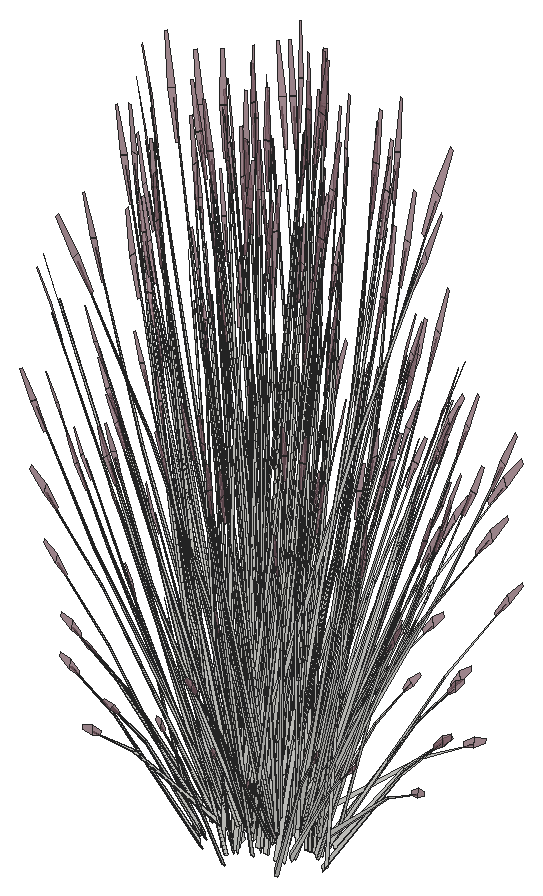
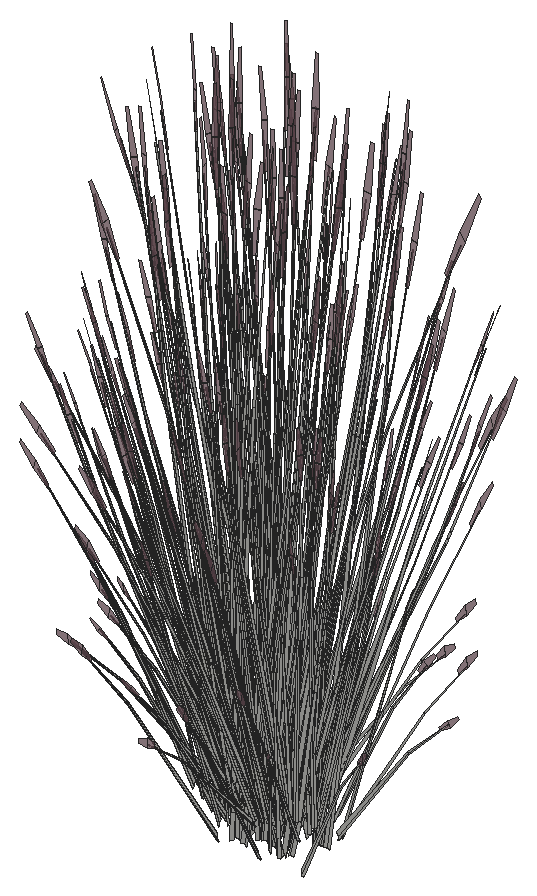
# SketchUp Ruby script. Lengths in inches.
U = 1.inch
M = Sketchup.active_model
def pt(a) = Geom::Point3d.new(a.map { |v| v * U })
def face(e, loops, mat)
  f = e.add_face(loops[0].map { |a| pt(a) })
  loops[1..].each { |l| e.add_face(l.map { |a| pt(a) }).erase! }
  f.material = f.back_material = mat if mat
  f
end
# faces: each face lists its corners as indices into pts; further lists are holes
def faces(e, pts, list, mat = nil) = list.each { |f| face(e, (f[0].is_a?(Array) ? f : [f]).map { |l| l.map { |i| pts[i] } }, mat) }
# xy, xz, yz: faces in a plane at the given z, y or x. An outline is a flat list of corners, or four numbers for a rectangle; further outlines are holes
def ring(l) = l.size == 4 ? [[l[0], l[1]], [l[2], l[1]], [l[2], l[3]], [l[0], l[3]]] : l.each_slice(2).to_a
def flat(e, list, mat, &to3) = list.each { |f| face(e, (f[0].is_a?(Array) ? f : [f]).map { |l| ring(l).map { |u, v| to3.(u, v) } }, mat) }
def xy(e, z, list, mat = nil) = flat(e, list, mat) { |x, y| [x, y, z] }
def xz(e, y, list, mat = nil) = flat(e, list, mat) { |x, z| [x, y, z] }
def yz(e, x, list, mat = nil) = flat(e, list, mat) { |y, z| [x, y, z] }
def lines(e, pts, list) = list.each { |a, b| e.add_line(pt(pts[a]), pt(pts[b])) }
# prism: a flat outline (further loops are holes) pulled along v
def prism(e, loops, v, mat = nil)
  f = face(e, loops, mat); d = Geom::Vector3d.new(v.map { |x| x * U })
  f.pushpull(f.normal.samedirection?(d) ? d.length : -d.length)
end
def box(e, o, s, mat = nil) = prism(e, [[o, [o[0] + s[0], o[1], o[2]], [o[0] + s[0], o[1] + s[1], o[2]], [o[0], o[1] + s[1], o[2]]]], [0, 0, s[2]], mat)
def at(x, y, z, deg = 0) = Geom::Transformation.translation(pt([x, y, z])) * Geom::Transformation.rotation(ORIGIN, Z_AXIS, deg.degrees)
def axes(o, x, y, z) = Geom::Transformation.new([*x, 0, *y, 0, *z, 0, *pt(o).to_a, 1])
def part(name) = M.definitions.add(name)
# library, detail: a bought-in or finely detailed component or shape, given as its bounding box
def library(name, o, s) = part(name).tap { |d| box(d.entities, o, s) }
def detail(e, o, s) = box(e.add_group.entities, o, s)
def put(e, d, t, mat = nil) = e.add_instance(d, t).tap { |i| i.material = mat if mat }
def group(e, t, mat = nil) = e.add_group.tap { |g| g.transformation = t; g.material = mat if mat }.entities
root = M.entities
M.materials.add("LightPink_Translucent").color = [144, 107, 117]
M.materials["LightPink_Translucent"].alpha = 0.75
c1 = part("blade")
p = [[2.15,0.21,22],[0,0.17,0],[0.09,0.45,0],[2.18,0.31,22],[2.29,0.31,22],[0.38,0.45,0],
  [2.48,0.24,33],[2.49,0.24,33],[2.48,0.22,33]]
faces(c1.entities,p,[[0,1,2,3],[4,5,2,3],[6,3,4,7],[8,0,3,6]])
c2 = part("seeds")
p = [[0.3,-0.1,1.38],[-0.01,-0.03,1.59],[-0.01,-0.03,0.03],[0.14,-0.07,-0.07],[0.29,-0.03,3],[0.15,0.01,3.11]]
faces(c2.entities,p,[[0,1,2,3],[1,0,4,5]],"LightPink_Translucent")
c3 = part("blade with seeds")
put(c3.entities,c1,at(0,0,0))
put(c3.entities,c2,axes([2.4,0.25,30.99],[1.5799,-0.05474,1.17369],[-0.12525,1.92788,0.29478],[-0.07173,-0.02425,1.56792]))
put(root,c3,axes([839.49,270.18,1.9375],[0.11478,-0.10046,0.85688],[0.28982,0.27117,0.06928],[-0.19878,0.12349,0.36631]))
put(root,c3,axes([838.8,270.44,2.26],[-0.40003,0.04673,-0.17707],[-0.10563,-0.26712,0.2286],[-0.11464,0.07175,0.4374]))
put(root,c3,axes([838.58,271.23,0.75],[0.06164,0.03267,0.88171],[0.10452,0.30266,-0.1347],[-0.13662,0.06454,0.15018]))
put(root,c3,axes([838.49,269.45,1.38],[0.2934,-0.0234,0.5743],[-0.18611,0.20614,0.42196],[-0.14499,-0.03092,0.12649]))
put(root,c3,axes([838.85,270.38,2.37],[-0.11397,-0.30091,0.24001],[0.44709,-0.05222,0.1979],[-0.13177,0.07077,0.49665]))
put(root,c3,axes([839.08,268.89,2.55],[0.37952,-0.24129,0.26881],[0.32731,0.25625,0.22165],[-0.17806,-0.04451,0.55625]))
put(root,c3,axes([838.76,270.33,2.37],[-0.31549,-0.13751,0.03215],[0.18368,-0.19581,0.2531],[-0.10115,0.06331,0.38595]))
put(root,c3,axes([839.4,270.43,1.9375],[0.08557,-0.11238,0.85688],[0.35897,0.23257,0.06928],[-0.16194,0.14495,0.36631]))
put(root,c3,axes([839.06,269.65,2.53],[0.38192,0.09121,0.17707],[-0.11139,0.2661,-0.2286],[-0.15377,0.0244,0.4374]))
put(root,c3,axes([839.125,270.47,2.34],[0.11806,0.29854,-0.25549],[-0.44709,0.05222,-0.1979],[-0.12812,0.08019,0.48886]))
put(root,c3,axes([839.25,268.89,2.37],[0.02314,-0.24862,0.03215],[0.34943,0.00682,0.2531],[-0.13385,-0.02602,0.38595]))
put(root,c3,axes([838.43,271.01,2.36],[-0.01142,0.0647,0.87472],[0.32418,0.22509,-0.13834],[-0.08487,0.10644,0.07015]))
put(root,c3,axes([840.24,270.26,1.03],[-0.47805,-0.0536,-0.31177],[0.10088,-0.33065,-0.08182],[-0.14266,-0.04007,0.68817]))
put(root,c3,axes([840.33,268.46,2.72],[-0.30671,0.31344,-0.0681],[-0.44417,-0.18058,-0.37797],[-0.1544,-0.08856,0.57432]))
put(root,c3,axes([839.49,269.07,2.53],[0.26148,0.20471,0.17707],[-0.29857,0.19378,-0.2286],[-0.1517,-0.02948,0.4374]))
put(root,c3,axes([840.19,268.71,2.49],[-0.39186,-0.15803,-0.35523],[0.27849,-0.27693,0.04287],[-0.14198,-0.09436,0.5025]))
put(root,c3,axes([840.01,268.72,2.34],[-0.45348,0.07772,-0.25549],[-0.07933,-0.29434,-0.1979],[-0.1218,-0.08435,0.48886]))
put(root,c3,axes([839.61,270.88,1.01],[-0.4301,-0.16348,-0.24825],[0.25708,-0.29314,0],[-0.09796,-0.03723,0.78752]))
put(root,c3,axes([839.43,268.45,0.75],[-0.04451,0.04307,0.88171],[-0.44986,0.09286,-0.1347],[-0.10868,-0.08448,0.15018]))
put(root,c3,axes([838.92,270.26,2.52],[0.4251,0.18028,-0.0608],[-0.24491,0.26108,-0.33747],[-0.1201,0.09075,0.51278]))
put(root,c3,axes([839.875,271.08,1.1875],[-0.28732,0.32763,0],[-0.4807,-0.18271,-0.25804],[-0.10948,-0.04161,0.81856]))
put(root,c3,axes([838.22,271.04,2.82],[0.40553,0.08728,-0.03244],[-0.12475,0.26862,-0.14708],[-0.06633,0.04078,0.48512]))
put(root,c3,axes([839.125,270.28,2.53],[0.40003,-0.04673,0.17707],[0.10563,0.26712,-0.2286],[-0.11464,0.07175,0.4374]))
put(root,c3,axes([839.35,271.56,1.3],[0.14502,-0.05158,0.71501],[0.35805,0.15552,-0.15377],[-0.10657,0.13457,0.3057]))
put(root,c3,axes([839.15,268.62,1.0625],[-0.13257,0.26698,-0.01946],[-0.40802,-0.08212,-0.08825],[-0.06195,-0.04367,0.29107]))
put(root,c3,axes([840.21,267.71,2.35],[-0.00857,0.03919,0.88692],[-0.42284,0.14223,-0.08381],[-0.12443,-0.0727,0.15695]))
put(root,c3,axes([839.76,268.28,1.3],[-0.02783,0.10696,0.71501],[-0.40683,0.08954,-0.15377],[-0.0951,-0.13825,0.3057]))
put(root,c3,axes([839.89,268.56,1.9375],[0.10505,0.10498,0.85688],[-0.48542,0.08838,0.06928],[-0.10971,-0.1648,0.36631]))
put(root,c3,axes([840.78,270.31,1.33],[-0.46399,0.21707,-0.14548],[-0.30855,-0.30672,-0.25001],[-0.11448,-0.03115,0.79854]))
put(root,c3,axes([839.5,270.99,2.37],[-0.32725,-0.22308,0.24001],[0.34753,-0.1924,0.1979],[-0.06036,0.10466,0.49665]))
put(root,c3,axes([840.06,268.5,2.26],[-0.07098,-0.26335,-0.17707],[0.40574,-0.06954,0.2286],[-0.10898,-0.07547,0.4374]))
put(root,c3,axes([838.93,269.83,1.1875],[-0.57465,0,0],[0,-0.36542,-0.25804],[0,-0.08323,0.81856]))
put(root,c3,axes([839.73,270.76,1.01],[-0.10795,-0.28489,-0.15489],[0.42874,-0.0809,0.15489],[-0.08643,-0.03285,0.69487]))
put(root,c3,axes([839.38,270.97,2.37],[-0.37765,-0.01523,0.03215],[0.01035,-0.23004,0.2531],[-0.03952,0.08812,0.38595]))
put(root,c3,axes([839.5,271.06,2.26],[-0.31095,0.17214,-0.17707],[-0.29435,-0.19656,0.2286],[-0.04479,0.09987,0.4374]))
put(root,c3,axes([841.09,270.54,1.03],[-0.30954,0.24575,-0.31177],[-0.38452,-0.22284,-0.08182],[-0.12404,0.0613,0.68817]))
put(root,c3,axes([840.3,268.72,2.53],[0.07098,0.26335,0.17707],[-0.40574,0.06954,-0.2286],[-0.10898,-0.07547,0.4374]))
put(root,c3,axes([838.39,271.67,2.35],[0.05214,-0.01974,0.88692],[0.43092,0.1313,-0.08381],[-0.01013,0.10932,0.15695]))
put(root,c3,axes([839.37,269.74,1.17],[-0.42746,0.27488,0.15378],[-0.42772,-0.27199,-0.18246],[-0.01493,-0.07806,0.82443]))
put(root,c3,axes([841.13,270.5,1.66],[0.39713,0.13184,0.7563],[-0.38905,0.28403,0.29908],[-0.17427,-0.16834,0.63403]))
put(root,c3,axes([839.62,268.11,1.38],[0.23972,0.1138,0.5743],[-0.34912,0.06841,0.42196],[-0.0747,-0.08746,0.12649]))
put(root,c3,axes([841.3,270.41,1.23],[-0.44875,-0.26316,-0.12596],[0.3776,-0.2955,0.27565],[-0.12084,0.03078,0.84108]))
put(root,c3,axes([840.49,270.15,1.11],[-0.27607,-0.27443,-0.2237],[0.41817,-0.19325,0.10766],[-0.08934,-0.03396,0.71822]))
put(root,c3,axes([839.71,270.88,2.67],[-0.01196,0.30243,-0.3943],[-0.50354,-0.02031,0.04758],[-0.05314,0.12813,0.55778]))
put(root,c3,axes([839.7,271.73,1.38],[-0.01189,-0.19441,0.5743],[0.29719,0.13866,0.42196],[-0.05845,0.09266,0.12649]))
put(root,c3,axes([840.12,268.41,2.55],[0.51193,-0.08404,0.26881],[0.08885,0.32966,0.22165],[-0.1204,-0.09716,0.55625]))
put(root,c3,axes([841.08,270.35,1.11],[-0.49904,0.02018,-0.2237],[-0.04513,-0.33504,0.10766],[-0.08934,0.03396,0.71822]))
put(root,c3,axes([840.23,268.48,2.37],[0.20887,-0.2077,0.03215],[0.29744,0.12092,0.2531],[-0.09616,-0.06659,0.38595]))
put(root,c3,axes([840.125,270.91,1.24],[0.4301,0.16348,0.24825],[-0.25708,0.29314,0],[-0.09796,-0.03723,0.78752]))
put(root,c3,axes([839.54,271.3,1.68],[0.0101,-0.16879,0.77173],[0.45413,0.08915,0.10664],[-0.03935,0.17989,0.36441]))
put(root,c3,axes([840.53,270.3125,1.22],[0.1218,-0.38743,-0.11714],[0.57753,0.06753,0.25635],[-0.10091,-0.0535,0.7822]))
put(root,c3,axes([840.74,270.4,1.31],[-0.08866,0.29179,0.0724],[-0.43315,-0.05065,-0.20674],[-0.07883,-0.02996,0.63372]))
put(root,c3,axes([840.69,267.86,2.36],[-0.07029,-0.04584,0.87472],[-0.46908,0.02906,-0.13834],[-0.07486,-0.10965,0.07015]))
put(root,c3,axes([841.6,271.22,1.01],[-0.4301,0.16348,-0.24825],[-0.25708,-0.29314,0],[-0.09796,0.03723,0.78752]))
put(root,c3,axes([839.06,269.59,1.01],[0,-0.32696,-0.24825],[0.51416,0,0],[0,-0.07447,0.78752]))
put(root,c3,axes([839.28,269.89,1.24],[0,0.32696,0.24825],[-0.51416,0,0],[0,-0.07447,0.78752]))
put(root,c3,axes([841.63,271.13,1.1],[-0.28374,-0.32877,-0.02571],[0.4807,-0.18271,0.25804],[-0.11845,0.0313,0.81815]))
put(root,c3,axes([839.81,270.98,2.5],[0.32898,0.21969,-0.2836],[-0.34753,0.1924,-0.21967],[-0.05006,0.11162,0.54264]))
put(root,c3,axes([841.5,271.09,1.01],[-0.42874,-0.0809,-0.15489],[0.10795,-0.28489,0.15489],[-0.08643,0.03285,0.69487]))
put(root,c3,axes([839.66,270.82,2.53],[0.31095,-0.17214,0.17707],[0.29435,0.19656,-0.2286],[-0.04479,0.09987,0.4374]))
put(root,c3,axes([840.4,269.96,1.33],[-0.51755,-0.15601,-0.14548],[0.2492,-0.32927,-0.25001],[-0.01626,-0.08084,0.79854]))
put(root,c3,axes([841.75,269.87,1.42],[-0.01255,-0.30784,0.70636],[0.56816,0.0798,0.29908],[-0.13438,0.16845,0.66675]))
put(root,c3,axes([839.47,270.86,2.7],[0.50507,0.0162,-0.06749],[-0.01381,0.30672,-0.3746],[-0.03508,0.11813,0.56919]))
put(root,c3,axes([839.45,271.31,1.41],[0.41748,-0.0579,0.03254],[0.09598,0.23326,-0.43152],[-0.02647,0.11808,0.3868]))
put(root,c3,axes([841.43,270.26,1.33],[0.05355,0.37308,-0.14548],[-0.55775,0.02256,-0.25001],[-0.09822,0.04969,0.79854]))
put(root,c3,axes([840.17,269.63,1.05],[-0.18873,-0.33528,-0.34918],[0.54365,-0.12075,-0.09164],[-0.02086,-0.11353,0.77075]))
put(root,c3,axes([841.4,268.57,2.52],[-0.44971,0.15222,-0.0608],[-0.221,-0.27017,-0.33747],[-0.05933,-0.11385,0.51278]))
put(root,c3,axes([841.02,268.58,2.34],[-0.45175,-0.08196,-0.25549],[0.15485,-0.28101,-0.1979],[-0.04142,-0.11314,0.48886]))
put(root,c3,axes([840.18,270.66,1.9375],[-0.01125,-0.12549,0.85688],[0.48751,0.08325,0.06928],[-0.03015,0.17883,0.36631]))
put(root,c3,axes([839.28,269.59,1.01],[0.32079,-0.20399,-0.15489],[0.32079,0.20399,0.15489],[0,-0.06571,0.69487]))
put(root,c3,axes([840.72,268.27,1.0625],[-0.31757,0.18757,-0.01946],[-0.29098,-0.20543,-0.08825],[-0.02049,-0.05821,0.29107]))
put(root,c3,axes([840.6,270.125,1.18],[0.58084,0.06889,0.22877],[-0.11821,0.38906,0.08977],[-0.08488,-0.03757,0.79428]))
put(root,c3,axes([840.45,270.05,1.36],[-0.22297,0.29461,0.2237],[-0.4633,-0.14179,-0.10766],[0,-0.06791,0.71822]))
put(root,c3,axes([841.18,268.63,2.49],[-0.21934,-0.26585,-0.35523],[0.45151,-0.14816,0.04287],[-0.05129,-0.12845,0.5025]))
put(root,c3,axes([840.28,270.75,1.24],[0.49383,-0.08678,0.08821],[0.12194,0.32295,0.17543],[-0.04404,-0.04705,0.80203]))
put(root,c3,axes([840.92,270.8,1.1],[-0.4633,-0.14679,0],[0.22297,-0.30501,0],[0,0,0.81353]))
put(root,c3,axes([841.27,268.67,2.53],[-0.13855,0.25143,0.17707],[-0.4042,-0.07334,-0.2286],[-0.03706,-0.10123,0.4374]))
put(root,c3,axes([841.99,271.16,1.1875],[0.28732,0.32763,0],[-0.4807,0.18271,-0.25804],[-0.10948,0.04161,0.81856]))
put(root,c3,axes([840.53,271.31,2.53],[-0.45283,-0.08548,0.26641],[0.15485,-0.28101,0.21967],[0.02721,0.11051,0.55128]))
put(root,c3,axes([840.41,271.33,2.37],[-0.33863,0.11112,0.03215],[-0.16575,-0.20263,0.2531],[0.0327,0.08932,0.38595]))
put(root,c3,axes([841.75,270.76,1.24],[0.13276,-0.32494,0.08821],[0.4858,0.09195,0.17543],[-0.08392,0.00158,0.80203]))
put(root,c3,axes([841.53,270.33,1.31],[0.33952,0.19644,0.0724],[-0.2832,0.22163,-0.20674],[-0.07883,0.02996,0.63372]))
put(root,c3,axes([841.41,270.09,1.15],[-0.42746,-0.28142,-0.03066],[0.42772,-0.28159,0],[-0.01493,-0.00983,0.87786]))
put(root,c3,axes([841.52,270.1875,1.36],[0.49904,-0.02018,0.2237],[0.04513,0.33504,-0.10766],[-0.08934,0.03396,0.71822]))
put(root,c3,axes([841.64,270.96,1.17],[0.57533,0.10627,0.15378],[-0.14394,0.37986,-0.18246],[-0.09522,0.04754,0.82443]))
put(root,c3,axes([840.8,268.04,0.75],[-0.07708,0.01178,0.88171],[-0.42627,-0.1326,-0.1347],[0.00715,-0.1106,0.15018]))
put(root,c3,axes([841.89,270.9375,1.24],[0.4301,-0.16348,0.24825],[0.25708,0.29314,0],[-0.09796,0.03723,0.78752]))
put(root,c3,axes([841.22,268.41,2.26],[0.13855,-0.25143,-0.17707],[0.4042,0.07334,0.2286],[-0.03706,-0.10123,0.4374]))
put(root,c3,axes([840.55,269.77,1.18],[0.1998,0.3656,0.22877],[-0.5709,0.12713,0.08977],[0.00698,-0.06718,0.79428]))
put(root,c3,axes([840.45,269.72,1.11],[0.22297,-0.29461,-0.2237],[0.4633,0.14179,0.10766],[0,-0.06791,0.71822]))
put(root,c3,axes([841.03,270.67,1.1],[-0.14994,-0.28188,0],[0.42817,-0.09871,0],[0,0,0.77185]))
put(root,c3,axes([840.48,271.26,0.75],[0.07437,-0.01779,0.88171],[0.44738,0.09793,-0.1347],[0.01308,0.11037,0.15018]))
put(root,c3,axes([840.58,271.36,2.26],[-0.13855,0.25143,-0.17707],[-0.4042,-0.07334,0.2286],[0.03706,0.10123,0.4374]))
put(root,c3,axes([841.63,270.11,1.11],[-0.22297,0.29461,-0.2237],[-0.4633,-0.14179,0.10766],[0,0.06791,0.71822]))
put(root,c3,axes([841.39,268.45,2.37],[0.33863,-0.11112,0.03215],[0.16575,0.20263,0.2531],[-0.0327,-0.08932,0.38595]))
put(root,c3,axes([840.29,271.81,2.36],[0.05825,0.05265,0.87472],[0.47011,0.02068,-0.13834],[0.04727,0.11612,0.07015]))
put(root,c3,axes([842.51,269.93,1.24],[-0.36107,-0.23816,0.08821],[0.36387,-0.231,0.17543],[-0.03988,0.04864,0.80203]))
put(root,c3,axes([841.27,269.8,1.1],[0,-0.37831,0],[0.57465,0,0],[0,0,0.89728]))
put(root,c3,axes([841.27,268.47,2.37],[0.45283,0.08548,0.24001],[-0.15485,0.28101,0.1979],[-0.02721,-0.11051,0.49665]))
put(root,c3,axes([840.73,269.87,1.22],[0.5178,0.15847,0.12032],[-0.2492,0.32927,0.25001],[0,-0.0759,0.80271]))
put(root,c3,axes([841.55,269.95,1.15],[0,0.37813,-0.02818],[-0.57465,0,0],[0,0.01188,0.89684]))
put(root,c3,axes([840.5625,269.65,1.36],[-0.49904,0.02018,0.2237],[-0.04513,-0.33504,-0.10766],[0.08934,-0.03396,0.71822]))
put(root,c3,axes([840.54,271.1,2.53],[0.13855,-0.25143,0.17707],[0.4042,0.07334,-0.2286],[0.03706,0.10123,0.4374]))
put(root,c3,axes([840.33,269.07,1.24],[-0.13276,0.32494,0.08821],[-0.4858,-0.09195,0.17543],[0.08392,-0.00158,0.80203]))
put(root,c3,axes([841.28,270.68,1.15],[0.1998,0.37562,-0.03006],[-0.5709,0.13162,0],[0.00698,0.01312,0.86086]))
put(root,c3,axes([840.09,268.67,1.1875],[-0.28732,-0.32763,0],[0.4807,-0.18271,-0.25804],[0.10948,-0.04161,0.81856]))
put(root,c3,axes([840.62,271.14,2.49],[0.21934,0.26585,-0.35523],[-0.45151,0.14816,0.04287],[0.05129,0.12845,0.5025]))
put(root,c3,axes([842.93,270.1875,1.1],[-0.57436,-0.00261,-0.02488],[0,-0.36542,0.24971],[-0.01805,0.08319,0.79176]))
put(root,c3,axes([841.8,269.09,1.24],[-0.49383,0.08678,0.08821],[-0.12194,-0.32295,0.17543],[0.04404,0.04705,0.80203]))
put(root,c3,axes([841.3,267.88,1.38],[0.05895,0.19066,0.5743],[-0.32704,-0.1056,0.42196],[0.03519,-0.09762,0.12649]))
put(root,c3,axes([841.08,272,2.82],[0.31757,-0.18757,-0.03244],[0.29098,0.20543,-0.14708],[0.02049,0.05821,0.48512]))
put(root,c3,axes([840.99,269.56,1.18],[-0.38104,0.29672,0.22877],[-0.45269,-0.26192,0.08977],[0.09186,-0.02961,0.79428]))
put(root,c3,axes([841.64,270.03,1.11],[0.32079,0.21119,0],[-0.32079,0.21119,0],[0,0,0.84633]))
put(root,c3,axes([841.64,269.78,1.36],[0.22297,-0.29461,0.2237],[0.4633,0.14179,-0.10766],[0,0.06791,0.71822]))
put(root,c3,axes([841.45,270.8,1.1],[0.4633,0.14679,0],[-0.22297,0.30501,0],[0,0,0.87477]))
put(root,c3,axes([840.79,271.19,2.34],[0.45175,0.08196,-0.25549],[-0.15485,0.28101,-0.1979],[0.04142,0.11314,0.48886]))
put(root,c3,axes([840.4,271.21,2.52],[0.44971,-0.15222,-0.0608],[0.221,0.27017,-0.33747],[0.05933,0.11385,0.51278]))
put(root,c3,axes([841.49,269.71,1.19],[-0.58084,-0.06889,0.24599],[0.11821,-0.38906,0.09653],[0.08488,0.03757,0.85407]))
put(root,c3,axes([842.7,268.1875,2.35],[-0.04667,0.02497,0.88692],[-0.45726,-0.08426,-0.08381],[-0.01655,-0.10898,0.15695]))
put(root,c3,axes([842.34,268.91,2.52],[-0.50507,-0.0162,-0.0608],[0.01381,-0.30672,-0.33747],[0.03508,-0.11813,0.51278]))
put(root,c3,axes([842.81,270.24,1.01],[-0.32079,0.20399,-0.15489],[-0.32079,-0.20399,0.15489],[0,0.06571,0.69487]))
put(root,c3,axes([841.89,270.2,1.05],[0.16851,0.29936,-0.34606],[-0.4854,0.10781,-0.09083],[0.01863,0.10137,0.76386]))
put(root,c3,axes([841.66,269.88,1.1],[0.51416,0,0],[0,0.33849,0],[0,0,0.89203]))
put(root,c3,axes([842.14,268.96,2.53],[-0.31095,0.17214,0.17707],[-0.29435,-0.19656,-0.2286],[0.04479,-0.09987,0.4374]))
put(root,c3,axes([841.16,269.51,1.36],[-0.27607,-0.27443,0.2237],[0.41817,-0.19325,-0.10766],[0.08934,0.03396,0.71822]))
put(root,c3,axes([840.66,269.57,1.33],[-0.05355,-0.37308,-0.14548],[0.55775,-0.02256,-0.25001],[0.09822,-0.04969,0.79854]))
put(root,c3,axes([841.83,269.85,1.31],[0.42817,-0.09535,0.0724],[0.14994,0.27228,-0.20674],[0,0.05992,0.63372]))
put(root,c3,axes([841.99,268.79,2.34],[-0.32898,-0.21969,-0.25549],[0.34753,-0.1924,-0.1979],[0.05006,-0.11162,0.48886]))
put(root,c3,axes([841.6875,269.87,1.33],[0.51755,0.15601,-0.14548],[-0.2492,0.32927,-0.25001],[0.01626,0.08084,0.79854]))
put(root,c3,axes([840.58,268.75,1.01],[0.42874,0.0809,-0.15489],[-0.10795,0.28489,0.15489],[0.08643,-0.03285,0.69487]))
put(root,c3,axes([841.78,268.4,1.3],[-0.13063,0.06618,0.71501],[-0.39122,-0.11583,-0.15377],[0.07252,-0.14406,0.3057]))
put(root,c3,axes([842.81,269.94,1.24],[0,-0.32696,0.24825],[0.51416,0,0],[0,0.07447,0.78752]))
put(root,c3,axes([843.03,270.25,1.01],[0,0.32696,-0.24825],[-0.51416,0,0],[0,0.07447,0.78752]))
put(root,c3,axes([841.66,271.24,2.37],[-0.45708,0.07503,0.24001],[-0.07933,-0.29434,0.1979],[0.1075,0.08675,0.49665]))
put(root,c3,axes([840.48,268.62,1.01],[0.4301,-0.16348,-0.24825],[0.25708,0.29314,0],[0.09796,-0.03723,0.78752]))
put(root,c3,axes([841.57,271.3,2.37],[-0.20887,0.2077,0.03215],[-0.29744,-0.12092,0.2531],[0.09616,0.06659,0.38595]))
put(root,c3,axes([841.04,270.61,1.9375],[-0.10505,-0.10498,0.85688],[0.48542,-0.08838,0.06928],[0.10971,0.1648,0.36631]))
put(root,c3,axes([841.35,269.43,1.31],[0.08866,-0.29179,0.0724],[0.43315,0.05065,-0.20674],[0.07883,0.02996,0.63372]))
put(root,c3,axes([841.96,268.92,1.24],[-0.4301,-0.16348,0.24825],[0.25708,-0.29314,0],[0.09796,0.03723,0.78752]))
put(root,c3,axes([842.1,268.89,2.49],[0.01196,-0.30243,-0.35523],[0.50354,0.02031,0.04287],[0.05314,-0.12813,0.5025]))
put(root,c3,axes([841.59,270.63,1.09],[0.48247,-0.11094,-0.09599],[0.16954,0.31956,0.00004],[0.05326,-0.01226,0.86949]))
put(root,c3,axes([841.51,271.06,2.53],[-0.07098,-0.26335,0.17707],[0.40574,-0.06954,-0.2286],[0.10898,0.07547,0.4374]))
put(root,c3,axes([841.6,269.68,1.11],[0.27607,0.27443,-0.2237],[-0.41817,0.19325,0.10766],[0.08934,0.03396,0.71822]))
put(root,c3,axes([841.78,269.54,2.24],[-0.39711,-0.16988,0.69141],[0.41931,-0.2645,0.29833],[0.12812,0.1594,0.66832]))
put(root,c3,axes([842.3,268.71,2.26],[0.31095,-0.17214,-0.17707],[0.29435,0.19656,0.2286],[0.04479,-0.09987,0.4374]))
put(root,c3,axes([841.11,271.43,2.35],[0.00136,-0.03958,0.88692],[0.39383,-0.17464,-0.08381],[0.1368,0.06234,0.15695]))
put(root,c3,axes([842.42,268.8,2.37],[0.37765,0.01523,0.03215],[-0.01035,0.23004,0.2531],[0.03952,-0.08812,0.38595]))
put(root,c3,axes([842.38,270.93,1.38],[-0.25875,-0.09401,0.5743],[0.33411,-0.09552,0.42196],[0.09012,0.08091,0.12649]))
put(root,c3,axes([841.46,270.83,1.3],[0.00811,-0.10838,0.71501],[0.38755,-0.12106,-0.15377],[0.11964,0.12972,0.3057]))
put(root,c3,axes([842.8,268.42,2.36],[-0.00444,-0.06507,0.87472],[-0.37468,-0.18807,-0.13834],[0.05793,-0.114,0.07015]))
put(root,c3,axes([840.99,269.29,1.03],[0.30954,-0.24575,-0.31177],[0.38452,0.22284,-0.08182],[0.12404,-0.0613,0.68817]))
put(root,c3,axes([842.3,268.78,2.37],[0.32725,0.22308,0.24001],[-0.34753,0.1924,0.1979],[0.06036,-0.10466,0.49665]))
put(root,c3,axes([842.35,269.07,1.01],[0.10795,0.28489,-0.15489],[-0.42874,0.0809,0.15489],[0.08643,0.03285,0.69487]))
put(root,c3,axes([843.16,270,1.1875],[0.57465,0,0],[0,0.36542,-0.25804],[0,0.08323,0.81856]))
put(root,c3,axes([841.3,269.53,1.33],[0.46399,-0.21707,-0.14548],[0.30855,0.30672,-0.25001],[0.11448,0.03115,0.79854]))
put(root,c3,axes([842.42,271.35,1.33],[-0.2947,-0.01025,0.5253],[0.19462,-0.21779,0.29003],[0.11642,0.07737,0.41205]))
put(root,c3,axes([842.68,269.49,2.53],[-0.40003,0.04673,0.17707],[-0.10563,-0.26712,-0.2286],[0.11464,-0.07175,0.4374]))
put(root,c3,axes([841.53,268.74,1.9375],[-0.08557,0.11238,0.85688],[-0.35897,-0.23257,0.06928],[0.16194,-0.14495,0.36631]))
put(root,c3,axes([841.47,271.19,2.52],[0.27385,-0.27986,-0.0608],[0.39658,0.16123,-0.33747],[0.13785,0.07907,0.51278]))
put(root,c3,axes([840.13,269.33,0.8],[-0.45234,0.1309,0.64464],[-0.14398,-0.37559,0.25048],[0.27777,0.00625,0.73321]))
put(root,c3,axes([842.89,269.51,2.52],[-0.4251,-0.18028,-0.0608],[0.24491,-0.26108,-0.33747],[0.1201,-0.09075,0.51278]))
put(root,c3,axes([841.79,271.06,2.34],[0.45348,-0.07772,-0.25549],[0.07933,0.29434,-0.1979],[0.1218,0.08435,0.48886]))
put(root,c3,axes([842.21,268.75,1.1875],[0.28732,-0.32763,0],[0.4807,0.18271,-0.25804],[0.10948,0.04161,0.81856]))
put(root,c3,axes([842.69,268.61,0.75],[-0.06878,-0.02576,0.88171],[-0.17668,-0.28776,-0.1347],[0.11919,-0.07809,0.15018]))
put(root,c3,axes([842.3125,270.7,2.53],[-0.26148,-0.20471,0.17707],[0.29857,-0.19378,-0.2286],[0.1517,0.02948,0.4374]))
put(root,c3,axes([842.47,268.95,1.01],[0.4301,0.16348,-0.24825],[-0.25708,0.29314,0],[0.09796,0.03723,0.78752]))
put(root,c3,axes([842.55,270.89,2.37],[-0.02314,0.24862,0.03215],[-0.34943,-0.00682,0.2531],[0.13385,0.02602,0.38595]))
put(root,c3,axes([842.45,271.27,0.75],[0.03348,-0.0472,0.88171],[0.42153,-0.13902,-0.1347],[0.12779,0.07195,0.15018]))
put(root,c3,axes([842.58,270.81,2.37],[-0.33886,0.21544,0.24001],[-0.29224,-0.22879,0.1979],[0.15898,0.03974,0.49665]))
put(root,c3,axes([842.68,269.3,2.34],[-0.11806,-0.29854,-0.25549],[0.44709,-0.05222,-0.1979],[0.12812,-0.08019,0.48886]))
put(root,c3,axes([843.46,270.84,1.96],[-0.08796,-0.27485,-0.01746],[0.41573,-0.06319,-0.07916],[0.08682,0.01742,0.26109]))
put(root,c3,axes([842.74,270.13,2.53],[-0.38192,-0.09121,0.17707],[0.11139,-0.2661,-0.2286],[0.15377,-0.0244,0.4374]))
put(root,c3,axes([841.84,269.58,1.03],[0.47805,0.0536,-0.31177],[-0.10088,0.33065,-0.08182],[0.14266,0.04007,0.68817]))
put(root,c3,axes([843.88,269.77,1.13],[-0.28491,-0.20907,-0.03244],[0.31204,-0.19157,-0.14708],[0.08842,-0.01349,0.48512]))
put(root,c3,axes([843.23,268.71,1.38],[-0.15307,0.16644,0.5743],[-0.13157,-0.22361,0.42196],[0.12643,-0.05603,0.12649]))
put(root,c3,axes([843.04,269.45,2.37],[0.31549,0.13751,0.03215],[-0.18368,0.19581,0.2531],[0.10115,-0.06331,0.38595]))
put(root,c3,axes([842.95,269.39,2.37],[0.11397,0.30091,0.24001],[-0.44709,0.05222,0.1979],[0.13177,-0.07077,0.49665]))
put(root,c3,axes([841.75,270.28,1.9375],[-0.1707,-0.05633,0.85688],[0.35326,-0.23632,0.06928],[0.22018,0.10661,0.36631]))
put(root,c3,axes([843.93,269.44,2.35],[-0.06002,-0.00248,0.88692],[-0.24926,-0.26607,-0.08381],[0.1001,-0.08748,0.15695]))
put(root,c3,axes([843.01,269.33,2.26],[0.40003,-0.04673,-0.17707],[0.10563,0.26712,0.2286],[0.11464,-0.07175,0.4374]))
put(root,c3,axes([842.6875,269.42,2.49],[0.24005,-0.25798,-0.35523],[0.42065,0.18334,0.04287],[0.14333,-0.09347,0.5025]))
put(root,c3,axes([843.09,270.21,2.37],[0.16879,0.22293,0.03215],[-0.30779,0.10912,0.2531],[0.13568,-0.02153,0.38595]))
put(root,c3,axes([842.68,270.81,2.26],[0.26148,0.20471,-0.17707],[-0.29857,0.19378,0.2286],[0.1517,0.02948,0.4374]))
put(root,c3,axes([842.39,270.83,2.52],[0.02461,-0.33251,-0.0608],[0.4659,0.00909,-0.33747],[0.17944,0.0231,0.51278]))
put(root,c3,axes([842.9,270.22,2.52],[-0.23123,-0.29606,-0.0608],[0.41039,-0.14549,-0.33747],[0.17294,-0.03906,0.51278]))
put(root,c3,axes([843.06,270.13,2.37],[-0.12984,0.29812,0.24001],[-0.42685,-0.10194,0.1979],[0.16786,-0.01792,0.49665]))
put(root,c3,axes([842.79,270.63,2.36],[0.09858,-0.00553,0.87472],[0.2704,-0.25401,-0.13834],[0.17535,0.03353,0.07015]))
put(root,c3,axes([842.88,269.96,2.34],[0.1245,-0.29741,-0.25549],[0.42685,0.10194,-0.1979],[0.17186,-0.02727,0.48886]))
put(root,c3,axes([843.96,270.15,1.38],[-0.28394,0.05398,0.5743],[0.13365,-0.22308,0.42196],[0.15063,0.01526,0.12649]))
put(root,c3,axes([843.04,269.18,1.3],[-0.16417,-0.00968,0.71501],[-0.16819,-0.25979,-0.15377],[0.20169,-0.07349,0.3057]))
put(root,c3,axes([843.15,270.1,2.26],[0.38192,0.09121,-0.17707],[-0.11139,0.2661,0.2286],[0.15377,-0.0244,0.4374]))
put(root,c3,axes([842.41,270.67,2.49],[0.45939,0.00787,-0.35523],[-0.03085,0.3315,0.04287],[0.19462,0.03498,0.5025]))
put(root,c3,axes([843.34,270.05,0.99],[-0.29599,0.03924,0.70792],[-0.04711,-0.31232,0.04052],[0.20731,-0.04727,0.40283]))
put(root,c3,axes([843.66,269.84,0.75],[-0.02402,-0.04964,0.88171],[0.16658,-0.29036,-0.1347],[0.16804,-0.00418,0.15018]))
put(root,c3,axes([843.82,271.1,2.35],[-0.04155,-0.02862,0.88692],[0.0909,-0.30682,-0.08381],[0.16368,-0.0196,0.15695]))
put(root,c3,axes([842.11,269.77,1.9375],[-0.19062,0.00741,0.85688],[0.12645,-0.32094,0.06928],[0.27165,0.01985,0.36631]))
put(root,c3,axes([842.8,270.07,2.49],[0.40382,-0.1444,-0.35523],[0.22505,0.29724,0.04287],[0.19512,-0.03377,0.5025]))
put(root,c3,axes([844.16,269.75,2.36],[0.06377,-0.0498,0.87472],[-0.08162,-0.30549,-0.13834],[0.16001,-0.05792,0.07015]))
put(root,c3,axes([843.42,270.51,1.3],[-0.11068,-0.08041,0.71501],[0.144,-0.26601,-0.15377],[0.22393,0.03604,0.3057]))
